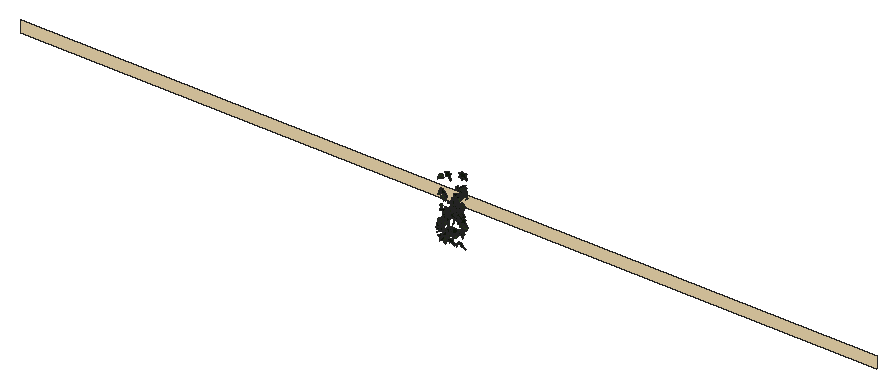
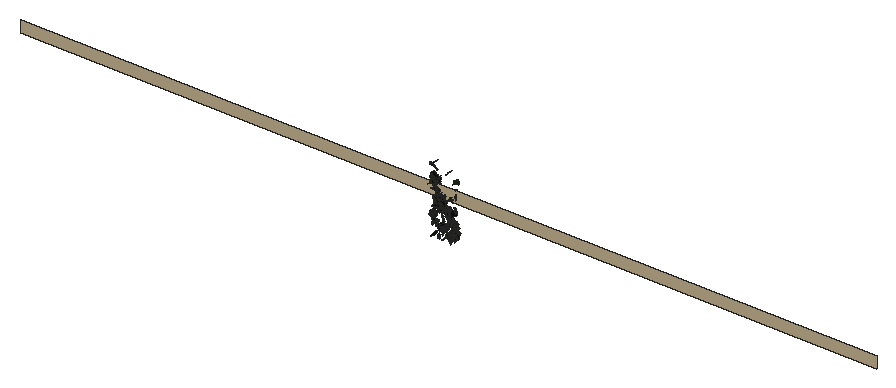
# SketchUp Ruby script. Lengths in inches.
U = 1.inch
M = Sketchup.active_model
def pt(a) = Geom::Point3d.new(a.map { |v| v * U })
def face(e, loops, mat)
  f = e.add_face(loops[0].map { |a| pt(a) })
  loops[1..].each { |l| e.add_face(l.map { |a| pt(a) }).erase! }
  f.material = f.back_material = mat if mat
  f
end
# faces: each face lists its corners as indices into pts; further lists are holes
def faces(e, pts, list, mat = nil) = list.each { |f| face(e, (f[0].is_a?(Array) ? f : [f]).map { |l| l.map { |i| pts[i] } }, mat) }
# xy, xz, yz: faces in a plane at the given z, y or x. An outline is a flat list of corners, or four numbers for a rectangle; further outlines are holes
def ring(l) = l.size == 4 ? [[l[0], l[1]], [l[2], l[1]], [l[2], l[3]], [l[0], l[3]]] : l.each_slice(2).to_a
def flat(e, list, mat, &to3) = list.each { |f| face(e, (f[0].is_a?(Array) ? f : [f]).map { |l| ring(l).map { |u, v| to3.(u, v) } }, mat) }
def xy(e, z, list, mat = nil) = flat(e, list, mat) { |x, y| [x, y, z] }
def xz(e, y, list, mat = nil) = flat(e, list, mat) { |x, z| [x, y, z] }
def yz(e, x, list, mat = nil) = flat(e, list, mat) { |y, z| [x, y, z] }
def lines(e, pts, list) = list.each { |a, b| e.add_line(pt(pts[a]), pt(pts[b])) }
# prism: a flat outline (further loops are holes) pulled along v
def prism(e, loops, v, mat = nil)
  f = face(e, loops, mat); d = Geom::Vector3d.new(v.map { |x| x * U })
  f.pushpull(f.normal.samedirection?(d) ? d.length : -d.length)
end
def box(e, o, s, mat = nil) = prism(e, [[o, [o[0] + s[0], o[1], o[2]], [o[0] + s[0], o[1] + s[1], o[2]], [o[0], o[1] + s[1], o[2]]]], [0, 0, s[2]], mat)
def at(x, y, z, deg = 0) = Geom::Transformation.translation(pt([x, y, z])) * Geom::Transformation.rotation(ORIGIN, Z_AXIS, deg.degrees)
def axes(o, x, y, z) = Geom::Transformation.new([*x, 0, *y, 0, *z, 0, *pt(o).to_a, 1])
def part(name) = M.definitions.add(name)
# library, detail: a bought-in or finely detailed component or shape, given as its bounding box
def library(name, o, s) = part(name).tap { |d| box(d.entities, o, s) }
def detail(e, o, s) = box(e.add_group.entities, o, s)
def put(e, d, t, mat = nil) = e.add_instance(d, t).tap { |i| i.material = mat if mat }
def group(e, t, mat = nil) = e.add_group.tap { |g| g.transformation = t; g.material = mat if mat }.entities
root = M.entities
M.materials.add("1026 AP 7946 SUNNY SIDE UP").color = [254, 231, 186]
M.materials.add("efeu1").color = [18, 25, 13]
M.materials.add("efeu2").color = [43, 57, 29]
c1 = part("ivyleaf_9")
p = [[1.54,2.16,1.25],[1.36,2.04,1.19],[-0.21,0.99,0.68],[-0.71,1.11,0.82],[-0.85,0.86,0.67],[-0.8,0.17,0.21],
  [-0.9,-0.01,0.1],[-0.67,-0.16,-0.02],[-0.08,-0.08,-0.05],[-0.03,-0.6,-0.4],[0.65,-0.88,-0.66],[0.83,-0.6,-0.49],
  [1.29,-0.42,-0.43],[1.8125,-0.07,-0.26],[1.21,0.44,0.15]]
faces(c1.entities,p,[[0,1,2,3,4,5,6,7,8,9,10,11,12,13,14]],"efeu1")
c2 = part("ivyleaf_10")
p = [[0,0.5,-0.03],[-0.0625,2.02,-0.43],[-0.19,2.01,-0.46],[-0.54,1.05,-0.29],[-0.52,0.625,-0.18],[-0.83,0.76,-0.28],
  [-1.16,0.64,-0.33],[-1.15,0.33,-0.24],[-0.77,-0.39,0.02],[-0.3,-0.51,0.16],[0.04,-0.48,0.23],[-0.02,2.01,-0.4375],
  [-0.06,2.01,-0.43],[0.04,-0.49,0.23],[0.67,-0.49,0.14],[1.38,0.36,-0.2],[1.375,0.51,-0.24],[0.81,0.65,-0.19],
  [0.62,0.59,-0.15],[0.6,1.09,-0.28],[0.5,1.23,-0.31]]
faces(c2.entities,p,[[0,1,2,3,4,5,6,7,8,9,10],[11,12,0,13,14,15,16,17,18,19,20]],"efeu2")
xz(root,213,[[29.75,274,177,276]],"1026 AP 7946 SUNNY SIDE UP")
put(root,c1,axes([102.26,212.91,269.98],[-0.38909,0.09409,-0.01702],[0.00603,-0.03752,-0.27074],[-0.15024,-0.24518,0.03321]),"1026 AP 7946 SUNNY SIDE UP")
put(root,c2,axes([102.07,212.85,275.0625],[-0.04177,-0.25771,-0.14632],[0.04767,0.13798,-0.2657],[0.45912,-0.03777,0.01427]),"1026 AP 7946 SUNNY SIDE UP")
put(root,c1,axes([102.23,212.68,269.12],[0.00018,0.2618,-0.01772],[-0.07293,-0.01838,-0.26557],[-0.40622,0.00341,0.04767]),"1026 AP 7946 SUNNY SIDE UP")
put(root,c2,axes([102.28,212.9,270.26],[-0.36396,-0.06711,0.12308],[-0.16337,-0.06809,-0.24638],[0.14129,-0.25161,0.03217]),"1026 AP 7946 SUNNY SIDE UP")
put(root,c2,axes([101.98,212.87,277.41],[-0.16539,-0.16217,-0.24308],[0.24264,0.17847,-0.19696],[0.3778,-0.18562,0.02008]),"1026 AP 7946 SUNNY SIDE UP")
put(root,c1,axes([101.97,212.875,269.98],[0.02729,-0.26526,-0.0416],[0.01272,0.03946,-0.27341],[0.42136,0.01599,0.01095]),"1026 AP 7946 SUNNY SIDE UP")
put(root,c2,axes([102.32,212.89,270.72],[0.33488,-0.00448,-0.17767],[-0.27056,-0.0248,-0.21842],[-0.01909,0.27291,-0.02116]),"1026 AP 7946 SUNNY SIDE UP")
put(root,c2,axes([102.18,212.87,275.79],[0.22941,-0.25653,0.03759],[0.01337,-0.03878,-0.30401],[0.40754,0.14567,-0.01119]),"1026 AP 7946 SUNNY SIDE UP")
put(root,c2,axes([102.13,212.94,270.33],[0.12289,0.25595,-0.03153],[-0.00312,-0.0329,-0.27578],[-0.40559,0.0778,-0.00743]),"1026 AP 7946 SUNNY SIDE UP")
put(root,c1,axes([102.3,212.93,269.93],[0.02948,0.26663,-0.02283],[0.00736,-0.02405,-0.27543],[-0.42084,0.01826,-0.00642]),"1026 AP 7946 SUNNY SIDE UP")
put(root,c1,axes([102.42,212.9375,269.77],[-0.38191,0.10456,-0.00559],[-0.00633,-0.02451,-0.27143],[-0.16456,-0.24172,0.02341]),"1026 AP 7946 SUNNY SIDE UP")
put(root,c2,axes([102.28,212.96,269.5],[-0.39792,0.07168,-0.01135],[0.00785,-0.02417,-0.27017],[-0.11387,-0.25217,0.02106]),"1026 AP 7946 SUNNY SIDE UP")
put(root,c2,axes([102.37,212.92,269.99],[-0.27576,0.19001,0.07625],[-0.1152,0.03088,-0.2642],[-0.29858,-0.18741,0.03152]),"1026 AP 7946 SUNNY SIDE UP")
put(root,c2,axes([102.38,212.86,270.75],[-0.26652,-0.21559,-0.00024],[0.01756,-0.01004,-0.28216],[0.33854,-0.1692,0.01445]),"1026 AP 7946 SUNNY SIDE UP")
put(root,c2,axes([102.34,212.86,270.16],[0.09375,-0.25699,0.05609],[0.03404,-0.05233,-0.27193],[0.41214,0.06278,0.0097]),"1026 AP 7946 SUNNY SIDE UP")
put(root,c2,axes([102.35,212.87,272.98],[0.28204,-0.21589,-0.0547],[0.00075,0.06707,-0.28543],[0.34913,0.17426,0.04481]),"1026 AP 7946 SUNNY SIDE UP")
put(root,c2,axes([102.4,212.93,270.3125],[0.09334,-0.26179,0.03156],[0.00372,-0.0324,-0.27668],[0.41471,0.05921,-0.00463]),"1026 AP 7946 SUNNY SIDE UP")
put(root,c1,axes([102.36,212.99,268.15],[-0.20361,-0.20172,0.09359],[0.00181,-0.10714,-0.24099],[0.3486,-0.11726,0.05591]),"1026 AP 7946 SUNNY SIDE UP")
put(root,c1,axes([102.5,212.89,270.42],[0.25417,0.18992,-0.09821],[-0.1309,-0.05507,-0.25587],[-0.30827,0.17998,0.02767]),"1026 AP 7946 SUNNY SIDE UP")
put(root,c2,axes([102.5,212.99,268.52],[0.09137,-0.25179,-0.01273],[0.00073,0.01132,-0.26613],[0.39629,0.05803,0.00343]),"1026 AP 7946 SUNNY SIDE UP")
put(root,c2,axes([102.52,212.99,269.01],[0.28481,-0.18347,-0.04422],[0.00715,0.06238,-0.26089],[0.29582,0.17513,0.04888]),"1026 AP 7946 SUNNY SIDE UP")
put(root,c1,axes([102.46,212.88,272.45],[0.36786,0.14363,-0.03281],[-0.02544,-0.03587,-0.28211],[-0.23021,0.23348,-0.02125]),"1026 AP 7946 SUNNY SIDE UP")
put(root,c2,axes([102.63,212.8125,270.98],[-0.23927,-0.22907,0.01036],[0.01839,-0.02136,-0.28256],[0.36017,-0.15109,0.02131]),"1026 AP 7946 SUNNY SIDE UP")
put(root,c1,axes([102.92,212.95,271.57],[-0.21962,0.23508,-0.02269],[0.00154,-0.02657,-0.28155],[-0.37145,-0.1391,0.01225]),"1026 AP 7946 SUNNY SIDE UP")
put(root,c2,axes([102.76,212.92,270.93],[-0.23027,-0.22985,-0.02207],[0.04911,0.00386,-0.27963],[0.35946,-0.14777,0.02407]),"1026 AP 7946 SUNNY SIDE UP")
put(root,c1,axes([102.59,212.88,268.0625],[0.08379,-0.24948,-0.02688],[-0.01627,0.02302,-0.26262],[0.39387,0.05403,-0.00513]),"1026 AP 7946 SUNNY SIDE UP")
put(root,c2,axes([102.85,212.91,274.52],[-0.33697,-0.18378,0.06857],[0.0064,-0.10438,-0.27963],[0.30784,-0.199,0.08088]),"1026 AP 7946 SUNNY SIDE UP")
put(root,c2,axes([102.75,212.93,270.69],[0.13253,0.25573,0.04118],[0.00379,0.03974,-0.27696],[-0.40662,0.08372,0.01084]),"1026 AP 7946 SUNNY SIDE UP")
put(root,c2,axes([102.875,212.99,269.39],[-0.02206,-0.26262,0.00196],[-0.01325,-0.00295,-0.27082],[0.41276,-0.01413,-0.00859]),"1026 AP 7946 SUNNY SIDE UP")
put(root,c1,axes([102.66,212.91,275.33],[0.10761,-0.28551,-0.01858],[-0.0048,0.01615,-0.30236],[0.44965,0.0685,0.00122]),"1026 AP 7946 SUNNY SIDE UP")
put(root,c2,axes([102.86,212.89,272.46],[0.2485,-0.23175,0.02667],[0.00651,-0.03006,-0.28882],[0.36685,0.15752,-0.01294]),"1026 AP 7946 SUNNY SIDE UP")
put(root,c2,axes([103.03,212.85,274.46],[0.28217,-0.2229,-0.05876],[-0.04211,0.04999,-0.29432],[0.35883,0.18115,0.01167]),"1026 AP 7946 SUNNY SIDE UP")
put(root,c2,axes([102.96,212.88,271.3],[0.42646,-0.04568,-0.00333],[-0.01186,-0.02696,-0.28204],[0.07099,0.26989,-0.0271]),"1026 AP 7946 SUNNY SIDE UP")
put(root,c1,axes([102.83,212.94,269.02],[0.10965,-0.2464,-0.06594],[0.04165,0.07161,-0.25952],[0.39757,0.06046,0.04538]),"1026 AP 7946 SUNNY SIDE UP")
put(root,c2,axes([103.12,212.95,270.72],[-0.25073,-0.20643,0.07114],[-0.01528,-0.08019,-0.26602],[0.34252,-0.15469,0.04021]),"1026 AP 7946 SUNNY SIDE UP")
put(root,c2,axes([103.09,212.99,269.15],[0.20356,-0.22378,-0.04288],[-0.0066,0.04407,-0.26541],[0.35748,0.12824,0.01952]),"1026 AP 7946 SUNNY SIDE UP")
put(root,c2,axes([103.0625,212.875,267.89],[-0.04258,-0.26003,0.01488],[0.10867,-0.0226,-0.25935],[0.39495,-0.02182,0.07297]),"1026 AP 7946 SUNNY SIDE UP")
put(root,c2,axes([103.18,212.86,272.84],[-0.38971,0.12654,0.02615],[-0.06148,-0.02286,-0.28413],[-0.19316,-0.24802,0.03769]),"1026 AP 7946 SUNNY SIDE UP")
put(root,c2,axes([103.07,212.96,271.18],[0.02314,0.27208,-0.00294],[0.00342,-0.00452,-0.28072],[-0.42786,0.01468,-0.0024]),"1026 AP 7946 SUNNY SIDE UP")
put(root,c1,axes([103.07,212.9375,271.49],[-0.08668,-0.26799,0.00907],[0.09693,-0.02292,-0.27394],[0.41041,-0.05118,0.06661]),"1026 AP 7946 SUNNY SIDE UP")
put(root,c2,axes([103.15,212.91,271.62],[0.2353,0.23113,-0.01275],[0.01164,-0.02106,-0.2832],[-0.36387,0.14879,-0.0173]),"1026 AP 7946 SUNNY SIDE UP")
put(root,c2,axes([103.21,212.79,268.35],[-0.10997,-0.23127,-0.11169],[0.1368,0.08273,-0.24207],[0.37668,-0.09756,0.05531]),"1026 AP 7946 SUNNY SIDE UP")
put(root,c1,axes([103.22,212.92,271.58],[-0.02655,-0.27553,-0.00385],[-0.00356,0.00231,-0.28436],[0.43324,-0.01687,-0.00257]),"1026 AP 7946 SUNNY SIDE UP")
put(root,c2,axes([103.29,212.95,271.97],[0.23313,-0.17407,0.16035],[0.12579,-0.13659,-0.23518],[0.34606,0.16691,-0.02254]),"1026 AP 7946 SUNNY SIDE UP")
put(root,c2,axes([103.46,212.97,268.71],[-0.1505,-0.23642,0.04592],[-0.00755,-0.04752,-0.26269],[0.37862,-0.09493,0.01301]),"1026 AP 7946 SUNNY SIDE UP")
put(root,c1,axes([103.69,212.96,272.36],[-0.42424,-0.0191,0.05988],[-0.08475,-0.05124,-0.27484],[0.04589,-0.27122,0.04606]),"1026 AP 7946 SUNNY SIDE UP")
put(root,c2,axes([103.52,212.84,270.67],[0.29559,-0.17844,-0.09822],[-0.04158,0.10602,-0.26028],[0.31464,0.18165,0.05788]),"1026 AP 7946 SUNNY SIDE UP")
put(root,c2,axes([103.39,212.94,271.92],[0.2836,0.18657,0.09928],[0.10222,0.06972,-0.26692],[-0.31317,0.19171,0.00279]),"1026 AP 7946 SUNNY SIDE UP")
put(root,c1,axes([103.375,212.88,278.27],[0.11707,-0.29256,-0.06105],[-0.00233,0.059,-0.31037],[0.46885,0.07334,0.0137]),"1026 AP 7946 SUNNY SIDE UP")
put(root,c2,axes([103.7,212.99,270.02],[-0.14885,-0.23252,0.08711],[-0.02458,-0.08615,-0.25854],[0.38897,-0.09442,0.017]),"1026 AP 7946 SUNNY SIDE UP")
put(root,c1,axes([103.76,212.92,272.55],[0.05537,0.27676,-0.0151],[-0.02474,-0.01434,-0.28715],[-0.43522,0.03603,0.0144]),"1026 AP 7946 SUNNY SIDE UP")
put(root,c1,axes([103.92,212.91,272.73],[-0.23185,0.23322,-0.05679],[-0.01524,-0.07199,-0.28075],[-0.377,-0.14052,0.04627]),"1026 AP 7946 SUNNY SIDE UP")
put(root,c1,axes([103.54,212.98,269.58],[0.22697,-0.21176,-0.0722],[-0.02257,0.07307,-0.26198],[0.34942,0.14227,0.02998]),"1026 AP 7946 SUNNY SIDE UP")
put(root,c1,axes([103.67,212.92,272.24],[-0.12847,-0.26698,-0.01305],[0.0068,0.01033,-0.28757],[0.42011,-0.08181,0.00067]),"1026 AP 7946 SUNNY SIDE UP")
put(root,c2,axes([103.77,212.95,272.44],[0.34046,-0.17472,-0.01642],[0.00422,0.02706,-0.28551],[0.2757,0.21535,0.02466]),"1026 AP 7946 SUNNY SIDE UP")
put(root,c2,axes([103.82,212.97,269.41],[0.11138,-0.24918,0.0418],[0.00373,-0.04295,-0.26695],[0.39732,0.07025,-0.00921]),"1026 AP 7946 SUNNY SIDE UP")
put(root,c2,axes([103.9,212.9,272.65],[-0.1415,-0.25881,0.06392],[0.00678,-0.06844,-0.28142],[0.41898,-0.0863,0.02614]),"1026 AP 7946 SUNNY SIDE UP")
put(root,c1,axes([103.77,212.92,272.4375],[-0.0522,-0.27829,0.00194],[-0.00044,-0.00345,-0.28874],[0.43762,-0.0332,-0.00006]),"1026 AP 7946 SUNNY SIDE UP")
put(root,c1,axes([103.72,212.85,269.77],[0.12521,-0.19925,-0.16167],[0.04687,0.16959,-0.20675],[0.39493,0.04304,0.07579]),"1026 AP 7946 SUNNY SIDE UP")
put(root,c1,axes([104.06,212.89,272.82],[0.02946,0.28016,0.02908],[-0.01153,0.02717,-0.28895],[-0.44236,0.01795,0.00947]),"1026 AP 7946 SUNNY SIDE UP")
put(root,c2,axes([103.87,212.96,272.94],[-0.40639,-0.03163,-0.11155],[0.17365,-0.0179,-0.2667],[0.03486,-0.27957,0.02803]),"1026 AP 7946 SUNNY SIDE UP")
put(root,c1,axes([103.76,212.95,268.15],[0.16286,-0.22239,-0.07829],[0.02686,0.08862,-0.24678],[0.36793,0.09197,0.05267]),"1026 AP 7946 SUNNY SIDE UP")
put(root,c2,axes([104,212.875,272.94],[0.32167,-0.19539,-0.00239],[-0.01954,-0.01126,-0.29099],[0.30662,0.20427,-0.01604]),"1026 AP 7946 SUNNY SIDE UP")
put(root,c2,axes([103.93,212.85,272.6875],[0.05424,0.26655,0.07493],[0.00262,0.07158,-0.27637],[-0.43383,0.03376,0.0077]),"1026 AP 7946 SUNNY SIDE UP")
put(root,c2,axes([104.03,212.86,274.44],[0.05585,-0.25291,-0.1348],[0.02111,0.13177,-0.26073],[0.44622,0.02542,0.02921]),"1026 AP 7946 SUNNY SIDE UP")
put(root,c2,axes([104.0625,212.92,272.93],[0.04514,-0.28107,0.00787],[-0.00004,-0.00928,-0.29112],[0.44219,0.02869,-0.00083]),"1026 AP 7946 SUNNY SIDE UP")
put(root,c2,axes([104.07,212.97,269.6],[0.00948,-0.2631,0.01316],[0.0005,-0.01427,-0.2712],[0.41431,0.00604,0.00003]),"1026 AP 7946 SUNNY SIDE UP")
put(root,c2,axes([104.14,212.91,273.03],[-0.25512,0.23168,-0.01117],[-0.04033,-0.03266,-0.28869],[-0.36255,-0.15939,0.03998]),"1026 AP 7946 SUNNY SIDE UP")
put(root,c2,axes([104.15,212.85,269.88],[0.1018,-0.24199,-0.09702],[0.03206,0.10011,-0.25369],[0.40626,0.05274,0.04433]),"1026 AP 7946 SUNNY SIDE UP")
put(root,c1,axes([103.97,212.9,273.18],[0.27882,-0.2134,0.06226],[0.07881,-0.03841,-0.28572],[0.34027,0.18376,0.01516]),"1026 AP 7946 SUNNY SIDE UP")
put(root,c1,axes([104.58,212.95,273.84],[-0.04006,0.02651,0.29085],[-0.44368,-0.02888,-0.02362],[0.0417,-0.28184,0.02809]),"1026 AP 7946 SUNNY SIDE UP")
put(root,c1,axes([104.1,212.79,272.27],[0.30435,-0.17805,-0.10921],[-0.05457,0.11381,-0.26407],[0.32041,0.18851,0.05876]),"1026 AP 7946 SUNNY SIDE UP")
put(root,c1,axes([104.47,212.92,273.59],[-0.06292,0.28216,-0.0179],[-0.001,-0.01926,-0.29368],[-0.44467,-0.03988,0.0032]),"1026 AP 7946 SUNNY SIDE UP")
put(root,c2,axes([104.3125,212.95,268.95],[0.16417,-0.22493,-0.08321],[0.03132,0.09468,-0.24851],[0.37381,0.09085,0.05736]),"1026 AP 7946 SUNNY SIDE UP")
put(root,c1,axes([104.18,212.85,269.6],[0.2066,-0.21805,-0.09733],[-0.01191,0.10268,-0.25778],[0.37271,0.12416,0.04571]),"1026 AP 7946 SUNNY SIDE UP")
put(root,c2,axes([104.42,212.97,271.14],[0.12488,-0.25862,-0.03835],[-0.01351,0.03476,-0.2785],[0.41031,0.07986,0.0025]),"1026 AP 7946 SUNNY SIDE UP")
put(root,c1,axes([104.17,212.96,273.04],[0.26011,-0.22751,-0.00021],[0.00186,-0.00048,-0.28979],[0.35774,0.16542,0.00166]),"1026 AP 7946 SUNNY SIDE UP")
put(root,c1,axes([104.4,212.9375,269.95],[-0.19435,-0.23647,-0.00697],[0.0161,0.00077,-0.27473],[0.37158,-0.12372,0.00826]),"1026 AP 7946 SUNNY SIDE UP")
put(root,c1,axes([104.76,212.89,274.38],[-0.40763,0.07925,0.10027],[-0.16221,-0.00908,-0.27677],[-0.11146,-0.2766,0.03606]),"1026 AP 7946 SUNNY SIDE UP")
put(root,c1,axes([104.48,212.96,274.15],[-0.23363,-0.24562,-0.00211],[0.01053,-0.00328,-0.29566],[0.38608,-0.14855,0.00678]),"1026 AP 7946 SUNNY SIDE UP")
put(root,c2,axes([104.64,212.97,269.3],[0.31687,-0.06933,-0.15784],[-0.20605,0.08417,-0.21687],[0.16483,0.2385,0.03234]),"1026 AP 7946 SUNNY SIDE UP")
put(root,c2,axes([104.51,212.97,269.1],[0.369,-0.11486,-0.0056],[-0.02196,-0.01768,-0.26831],[0.17942,0.23405,-0.02131]),"1026 AP 7946 SUNNY SIDE UP")
put(root,c1,axes([104.37,212.81,272.32],[0.11073,-0.25304,-0.11169],[-0.01871,0.10753,-0.26946],[0.43158,0.06959,0.01697]),"1026 AP 7946 SUNNY SIDE UP")
put(root,c2,axes([104.62,212.91,273.9],[-0.11425,-0.27692,0.02063],[0.00777,-0.02362,-0.29487],[0.43669,-0.07203,0.01065]),"1026 AP 7946 SUNNY SIDE UP")
put(root,c2,axes([104.63,212.98,272.15],[-0.29183,-0.19027,0.07573],[0.01014,-0.10616,-0.26307],[0.32119,-0.16952,0.07711]),"1026 AP 7946 SUNNY SIDE UP")
put(root,c2,axes([104.7,212.75,269.08],[0.39988,0.03924,0.10711],[-0.16695,0.01099,0.26389],[0.05049,-0.27444,0.02425]),"1026 AP 7946 SUNNY SIDE UP")
put(root,c2,axes([104.72,212.78,269.66],[-0.09667,-0.25283,-0.05976],[0.03017,0.05354,-0.26767],[0.40626,-0.06414,0.00566]),"1026 AP 7946 SUNNY SIDE UP")
put(root,c2,axes([104.77,212.82,274.53],[-0.38217,0.15651,0.00629],[-0.02535,-0.01543,-0.29706],[-0.24493,-0.24262,0.02094]),"1026 AP 7946 SUNNY SIDE UP")
put(root,c2,axes([104.83,212.86,269.49],[-0.26797,-0.19269,0.06087],[-0.02506,-0.06567,-0.2635],[0.31644,-0.16838,0.03068]),"1026 AP 7946 SUNNY SIDE UP")
put(root,c1,axes([104.86,212.86,269.6],[0.13664,0.25553,0.01766],[-0.00113,0.01681,-0.27788],[-0.40255,0.08669,0.00678]),"1026 AP 7946 SUNNY SIDE UP")
put(root,c1,axes([104.65,212.81,270.06],[0.09388,-0.23897,-0.10666],[0.02257,0.10771,-0.25025],[0.40805,0.04902,0.03838]),"1026 AP 7946 SUNNY SIDE UP")
put(root,c2,axes([105.14,212.75,273.82],[-0.17748,0.07725,0.26498],[-0.40264,0.05163,-0.13166],[-0.12512,-0.2757,0.04779]),"1026 AP 7946 SUNNY SIDE UP")
put(root,c2,axes([104.9,212.92,274.33],[0.27935,-0.22157,-0.05583],[0.01193,0.07284,-0.28746],[0.358,0.17046,0.05314]),"1026 AP 7946 SUNNY SIDE UP")
put(root,c1,axes([104.66,212.89,274.92],[0.25517,-0.24311,0.01806],[0.02187,-0.01346,-0.30117],[0.3828,0.16282,0.00516]),"1026 AP 7946 SUNNY SIDE UP")
put(root,c1,axes([104.84,212.93,274.3],[-0.18918,-0.17114,-0.20607],[0.19854,0.15425,-0.21434],[0.36189,-0.17409,0.00987]),"1026 AP 7946 SUNNY SIDE UP")
put(root,c1,axes([104.89,212.89,274.42],[-0.12628,-0.25688,-0.10686],[0.10945,0.08428,-0.27391],[0.42075,-0.09902,0.03918]),"1026 AP 7946 SUNNY SIDE UP")
put(root,c2,axes([105.07,213,268.07],[0.00428,-0.2461,0.07031],[0.00218,-0.06963,-0.25395],[0.40216,0.003,0.00063]),"1026 AP 7946 SUNNY SIDE UP")
put(root,c1,axes([104.83,212.93,274.23],[0.1924,-0.25785,0.03857],[0.02502,-0.03551,-0.29423],[0.40927,0.12339,-0.00015]),"1026 AP 7946 SUNNY SIDE UP")
put(root,c1,axes([104.76,212.88,274.1],[0.3787,-0.13031,0.08514],[0.09715,-0.06044,-0.28148],[0.22303,0.2476,-0.02197]),"1026 AP 7946 SUNNY SIDE UP")
put(root,c2,axes([105.18,212.92,275.25],[-0.22453,-0.24306,0.07649],[-0.03806,-0.07336,-0.29039],[0.39844,-0.14397,0.01537]),"1026 AP 7946 SUNNY SIDE UP")
put(root,c1,axes([104.95,212.76,275.65],[0.39327,0.15079,0.04254],[0.07038,0.0039,-0.30016],[-0.23517,0.25333,-0.01869]),"1026 AP 7946 SUNNY SIDE UP")
put(root,c1,axes([104.93,213.01,272.76],[0.19339,-0.24869,-0.02099],[0.00445,0.02253,-0.28539],[0.39214,0.12239,0.01359]),"1026 AP 7946 SUNNY SIDE UP")
put(root,c1,axes([105.08,212.99,274.92],[-0.1269,-0.27659,0.01621],[-0.00036,-0.01796,-0.29689],[0.43576,-0.08056,0.00448]),"1026 AP 7946 SUNNY SIDE UP")
put(root,c1,axes([105,212.9,274],[0.07111,-0.2794,-0.02671],[0.00972,0.02565,-0.29124],[0.44088,0.0445,0.01073]),"1026 AP 7946 SUNNY SIDE UP")
put(root,c1,axes([105.01,212.87,273.72],[0.16504,-0.25809,-0.06026],[-0.01047,0.05876,-0.28623],[0.41547,0.104,0.01672]),"1026 AP 7946 SUNNY SIDE UP")
put(root,c1,axes([105.03,212.99,272.03],[0.12673,-0.2633,-0.00721],[-0.00073,0.00562,-0.28364],[0.4141,0.08059,0.00171]),"1026 AP 7946 SUNNY SIDE UP")
put(root,c1,axes([105.05,212.89,274.6875],[0.33371,-0.1984,-0.01598],[-0.03284,-0.0013,-0.2989],[0.31106,0.21271,-0.01441]),"1026 AP 7946 SUNNY SIDE UP")
put(root,c1,axes([104.99,212.79,276.48],[0.37656,-0.16202,0.06185],[0.09726,-0.0171,-0.29725],[0.25422,0.24653,0.0221]),"1026 AP 7946 SUNNY SIDE UP")
put(root,c1,axes([105.44,212.95,275.375],[0.0314,0.28843,-0.03212],[-0.02841,-0.03159,-0.29759],[-0.45556,0.02185,0.01635]),"1026 AP 7946 SUNNY SIDE UP")
put(root,c1,axes([105.13,212.89,272.48],[0.14194,-0.28778,-0.0192],[-0.0129,0.01524,-0.31061],[0.45312,0.09058,-0.00283]),"1026 AP 7946 SUNNY SIDE UP")
put(root,c1,axes([105.15,212.93,273.21],[0.18739,-0.25456,-0.02326],[-0.01673,0.01836,-0.28945],[0.40131,0.11963,-0.0012]),"1026 AP 7946 SUNNY SIDE UP")
put(root,c1,axes([105.59,212.9,275.6],[-0.13575,0.27897,-0.03948],[-0.0071,-0.0431,-0.30059],[-0.44306,-0.08479,0.01691]),"1026 AP 7946 SUNNY SIDE UP")
put(root,c1,axes([105.17,212.82,276.74],[0.26501,-0.24736,-0.04864],[-0.02639,0.04396,-0.3079],[0.39468,0.16903,0.01207]),"1026 AP 7946 SUNNY SIDE UP")
put(root,c2,axes([105.37,212.92,275.21],[0.30835,0.21718,-0.01309],[-0.03175,-0.00053,-0.30108],[-0.34073,0.1966,0.0162]),"1026 AP 7946 SUNNY SIDE UP")
put(root,c1,axes([105.35,212.93,271.36],[0.13572,-0.25854,0.03251],[0.00317,-0.03413,-0.28085],[0.40983,0.08589,-0.0086]),"1026 AP 7946 SUNNY SIDE UP")
put(root,c1,axes([105.71,212.84,270.28],[0.06265,0.2619,0.07378],[-0.04289,0.07439,-0.26982],[-0.42416,0.03116,0.03818]),"1026 AP 7946 SUNNY SIDE UP")
put(root,c2,axes([105.64,212.9,275.65],[-0.23804,0.2501,0.04176],[-0.05419,0.02479,-0.30055],[-0.39434,-0.15438,0.01609]),"1026 AP 7946 SUNNY SIDE UP")
put(root,c2,axes([105.46,212.66,270.05],[0.05669,-0.08686,-0.26572],[0.27064,0.20824,-0.04633],[0.33056,-0.1556,0.0835]),"1026 AP 7946 SUNNY SIDE UP")
put(root,c1,axes([105.71,212.83,275.92],[0.19358,0.25657,0.071],[-0.00145,0.07479,-0.29084],[-0.41715,0.1188,0.03396]),"1026 AP 7946 SUNNY SIDE UP")
put(root,c1,axes([105.43,212.91,275.63],[0.44146,-0.0813,0.01722],[0.02268,-0.01193,-0.30109],[0.12867,0.28103,-0.00601]),"1026 AP 7946 SUNNY SIDE UP")
put(root,c1,axes([105.63,212.99,272.63],[-0.15343,-0.25925,-0.0234],[0.01147,0.01995,-0.28525],[0.40885,-0.09785,-0.00078]),"1026 AP 7946 SUNNY SIDE UP")
put(root,c1,axes([105.9,212.92,276.1],[-0.10848,0.28638,-0.0291],[0.00674,-0.02969,-0.30363],[-0.4527,-0.06906,0.00245]),"1026 AP 7946 SUNNY SIDE UP")
put(root,c1,axes([106.01,212.93,277],[-0.26365,0.2454,-0.03084],[0.00587,-0.03533,-0.30591],[-0.38895,-0.16688,0.01628]),"1026 AP 7946 SUNNY SIDE UP")
put(root,c1,axes([105.73,212.96,269.91],[-0.02384,-0.26652,0.00871],[-0.00145,-0.00994,-0.27507],[0.41937,-0.01519,-0.00045]),"1026 AP 7946 SUNNY SIDE UP")
put(root,c1,axes([105.67,212.83,268.21],[0.30029,-0.16098,-0.08504],[-0.07116,0.07235,-0.25561],[0.27475,0.19468,0.02675]),"1026 AP 7946 SUNNY SIDE UP")
put(root,c2,axes([105.91,212.86,273.13],[0.03832,-0.27927,0.01018],[-0.00327,-0.01169,-0.28884],[0.43948,0.02426,-0.00303]),"1026 AP 7946 SUNNY SIDE UP")
put(root,c1,axes([106.19,212.95,278.71],[-0.27025,0.24414,0.06788],[-0.09184,0.03747,-0.30624],[-0.38629,-0.17971,0.02532]),"1026 AP 7946 SUNNY SIDE UP")
put(root,c1,axes([105.87,212.66,277.0625],[0.19661,0.22994,0.15413],[0.10187,0.13354,-0.26879],[-0.418,0.1407,0.00699]),"1026 AP 7946 SUNNY SIDE UP")
put(root,c2,axes([106,212.875,276.39],[0.21884,-0.24658,-0.08478],[0.01746,0.09737,-0.28551],[0.40769,0.12819,0.05774]),"1026 AP 7946 SUNNY SIDE UP")
put(root,c1,axes([105.82,212.96,271.94],[0.10663,-0.23971,-0.12172],[0.01278,0.12231,-0.25304],[0.41908,0.05726,0.03869]),"1026 AP 7946 SUNNY SIDE UP")
put(root,c2,axes([105.99,212.78,271.34],[-0.14831,-0.25612,-0.12832],[0.11263,0.10409,-0.27903],[0.4324,-0.11496,0.02867]),"1026 AP 7946 SUNNY SIDE UP")
put(root,c2,axes([106.07,213,271.0625],[-0.36527,-0.13814,-0.01217],[0.0298,-0.01035,-0.27783],[0.21585,-0.23233,0.01777]),"1026 AP 7946 SUNNY SIDE UP")
put(root,c2,axes([106.08,212.84,269.97],[-0.01207,-0.23382,-0.13679],[0.02073,0.13102,-0.24011],[0.42126,-0.01315,0.00789]),"1026 AP 7946 SUNNY SIDE UP")
put(root,c2,axes([106.07,212.91,276.49],[-0.34354,0.20128,-0.00726],[-0.03584,-0.03671,-0.30311],[-0.31473,-0.21553,0.04244]),"1026 AP 7946 SUNNY SIDE UP")
put(root,c1,axes([105.8,212.83,279.1],[0.20617,-0.2694,-0.09115],[0.04022,0.1067,-0.30023],[0.4433,0.11561,0.06963]),"1026 AP 7946 SUNNY SIDE UP")
put(root,c2,axes([106.07,212.8,274.35],[0.32853,-0.18381,-0.08117],[-0.03109,0.09294,-0.28056],[0.31228,0.20263,0.05746]),"1026 AP 7946 SUNNY SIDE UP")
put(root,c2,axes([106.16,212.84,276.9],[-0.29915,-0.2218,-0.06536],[0.07396,0.04155,-0.30067],[0.35458,-0.1958,0.00757]),"1026 AP 7946 SUNNY SIDE UP")
put(root,c2,axes([106.11,212.9,276.71],[0.4604,-0.05276,-0.0141],[-0.00787,0.04683,-0.30268],[0.08522,0.28934,0.04821]),"1026 AP 7946 SUNNY SIDE UP")
put(root,c2,axes([106.24,212.83,274.05],[0.23045,-0.21092,-0.12742],[-0.05516,0.12318,-0.26105],[0.37953,0.14598,0.03943]),"1026 AP 7946 SUNNY SIDE UP")
put(root,c2,axes([106.35,212.93,270.96],[0.28691,0.05931,-0.1982],[-0.28137,-0.07219,-0.19784],[-0.14617,0.25539,-0.0082]),"1026 AP 7946 SUNNY SIDE UP")
put(root,c2,axes([106.18,212.89,271.12],[0.24023,-0.21563,0.06967],[0.0475,-0.0629,-0.27237],[0.35274,0.15532,-0.01077]),"1026 AP 7946 SUNNY SIDE UP")
put(root,c1,axes([106,212.96,276.18],[0.21589,-0.2352,-0.11912],[-0.00589,0.12731,-0.27378],[0.41114,0.12533,0.05863]),"1026 AP 7946 SUNNY SIDE UP")
put(root,c2,axes([106.31,212.95,276.12],[-0.09799,-0.28043,0.06508],[0.00088,-0.06639,-0.29596],[0.45256,-0.06059,0.01467]),"1026 AP 7946 SUNNY SIDE UP")
